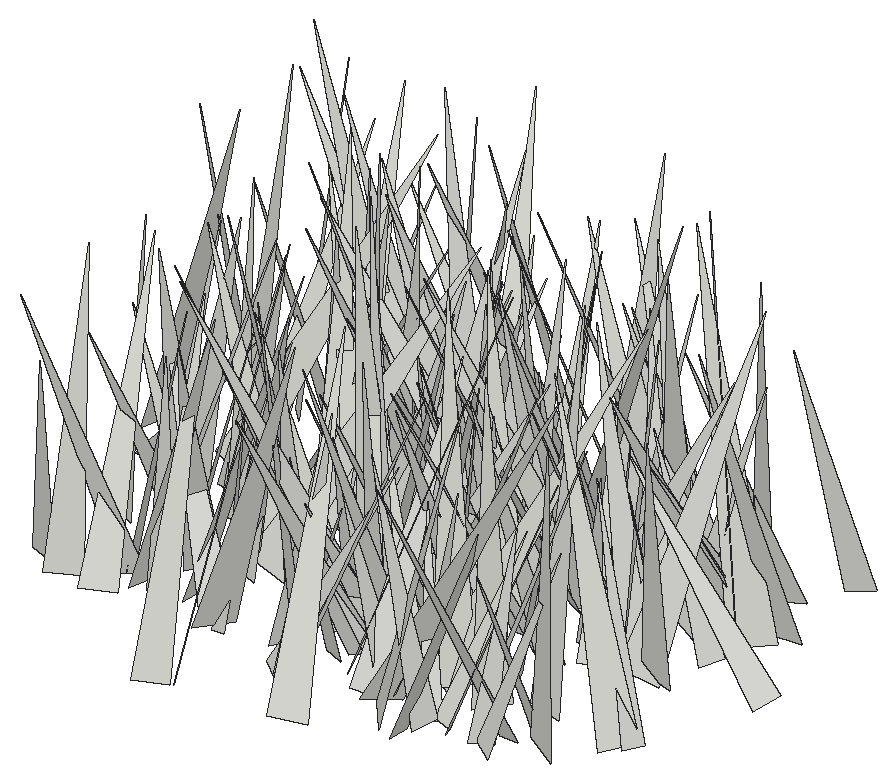
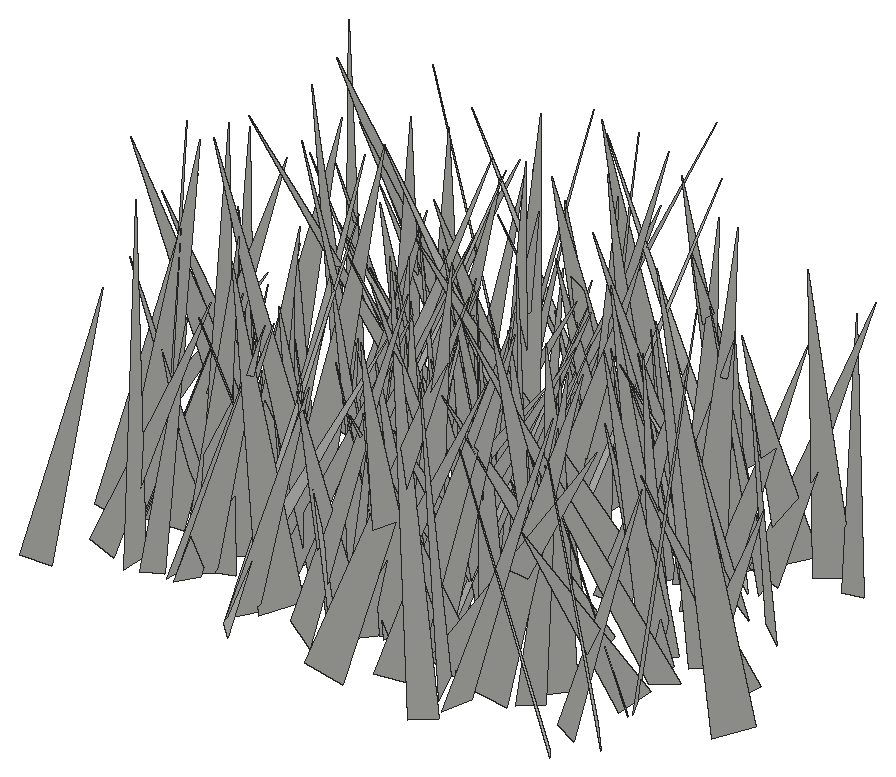
# SketchUp Ruby script. Lengths in inches.
U = 1.inch
M = Sketchup.active_model
def pt(a) = Geom::Point3d.new(a.map { |v| v * U })
def face(e, loops, mat)
  f = e.add_face(loops[0].map { |a| pt(a) })
  loops[1..].each { |l| e.add_face(l.map { |a| pt(a) }).erase! }
  f.material = f.back_material = mat if mat
  f
end
# faces: each face lists its corners as indices into pts; further lists are holes
def faces(e, pts, list, mat = nil) = list.each { |f| face(e, (f[0].is_a?(Array) ? f : [f]).map { |l| l.map { |i| pts[i] } }, mat) }
# xy, xz, yz: faces in a plane at the given z, y or x. An outline is a flat list of corners, or four numbers for a rectangle; further outlines are holes
def ring(l) = l.size == 4 ? [[l[0], l[1]], [l[2], l[1]], [l[2], l[3]], [l[0], l[3]]] : l.each_slice(2).to_a
def flat(e, list, mat, &to3) = list.each { |f| face(e, (f[0].is_a?(Array) ? f : [f]).map { |l| ring(l).map { |u, v| to3.(u, v) } }, mat) }
def xy(e, z, list, mat = nil) = flat(e, list, mat) { |x, y| [x, y, z] }
def xz(e, y, list, mat = nil) = flat(e, list, mat) { |x, z| [x, y, z] }
def yz(e, x, list, mat = nil) = flat(e, list, mat) { |y, z| [x, y, z] }
def lines(e, pts, list) = list.each { |a, b| e.add_line(pt(pts[a]), pt(pts[b])) }
# prism: a flat outline (further loops are holes) pulled along v
def prism(e, loops, v, mat = nil)
  f = face(e, loops, mat); d = Geom::Vector3d.new(v.map { |x| x * U })
  f.pushpull(f.normal.samedirection?(d) ? d.length : -d.length)
end
def box(e, o, s, mat = nil) = prism(e, [[o, [o[0] + s[0], o[1], o[2]], [o[0] + s[0], o[1] + s[1], o[2]], [o[0], o[1] + s[1], o[2]]]], [0, 0, s[2]], mat)
def at(x, y, z, deg = 0) = Geom::Transformation.translation(pt([x, y, z])) * Geom::Transformation.rotation(ORIGIN, Z_AXIS, deg.degrees)
def axes(o, x, y, z) = Geom::Transformation.new([*x, 0, *y, 0, *z, 0, *pt(o).to_a, 1])
def part(name) = M.definitions.add(name)
# library, detail: a bought-in or finely detailed component or shape, given as its bounding box
def library(name, o, s) = part(name).tap { |d| box(d.entities, o, s) }
def detail(e, o, s) = box(e.add_group.entities, o, s)
def put(e, d, t, mat = nil) = e.add_instance(d, t).tap { |i| i.material = mat if mat }
def group(e, t, mat = nil) = e.add_group.tap { |g| g.transformation = t; g.material = mat if mat }.entities
root = M.entities
c1 = part("fur_instance\#9")
p = [[0.8125,0,1.79],[0.67,-0.02,1.48],[0,-0.11,0],[0,0.11,0]]
faces(c1.entities,p,[[0,1,2,3]])
put(root,c1,axes([121.09,24.84,-27.1],[-5.92228,3.52878,0.304],[3.26745,5.67188,-2.1844],[1.36692,1.73077,6.53866]))
put(root,c1,axes([125.08,27.3125,-27.1],[6.15209,3.35933,0.33959],[3.37614,-6.1107,-0.71393],[0.04606,-0.78923,6.97306]))
put(root,c1,axes([133.24,29.44,-27.1],[-1.88046,-5.21634,0.33238],[-5.10911,1.75978,-1.28722],[-1.10347,0.74146,5.39346]))
put(root,c1,axes([128.65,27.92,-27.1],[5.36031,4.39922,1.5205],[4.6383,-5.24227,-1.18439],[-0.38885,-1.88772,6.83252]))
put(root,c1,axes([130.35,28.41,-27.1],[-5.09295,0.86723,1.4086],[1.03106,5.23004,0.50795],[1.29351,-0.75432,5.14123]))
put(root,c1,axes([121.52,25.7,-27.1],[6.37842,4.90538,1.53696],[4.59516,-6.53882,1.79932],[-2.30422,0.53885,7.84279]))
put(root,c1,axes([126.4375,25.72,-27.1],[-1.83957,6.80237,0.25254],[6.80704,1.83779,0.08208],[-0.01336,-0.2652,7.04624]))
put(root,c1,axes([112.64,29.51,-27.1],[-0.50328,-4.91347,1.0032],[-4.85841,0.72759,1.12622],[1.24277,0.85458,4.80907]))
put(root,c1,axes([120.26,29.36,-27.1],[6.42408,-3.63909,0.41323],[-3.66082,-6.40525,0.50369],[-0.11006,0.64215,7.36601]))
put(root,c1,axes([134.57,29.54,-27.1],[-2.31612,-6.1908,2.36322],[-6.27799,2.85121,1.3163],[2.12077,1.67923,6.47748]))
put(root,c1,axes([123.97,27.97,-27.1],[2.98745,4.37857,0.43851],[4.21633,-2.69647,-1.80015],[1.25963,-1.35874,4.98559]))
put(root,c1,axes([133,28.26,-27.1],[2.35379,3.88662,0.95748],[3.9563,-2.09005,-1.24191],[0.60851,-1.44527,4.3708]))
put(root,c1,axes([124.41,28.4,-27.1],[4.29417,-2.87763,1.75823],[-3.19183,-4.38696,0.6155],[-1.08829,1.5119,5.13243]))
put(root,c1,axes([124.15,29.3,-27.1],[-6.04607,-3.24149,2.31572],[-3.3744,6.40425,0.15438],[2.11738,0.95032,6.85845]))
put(root,c1,axes([125.6,31.08,-27.1],[1.43774,-5.64122,0.58152],[-5.34924,-1.54822,-1.79367],[-1.88339,0.09091,5.53834]))
put(root,c1,axes([133.97,30.2,-27.1],[-1.2303,-3.6424,0.32202],[-3.65502,1.23499,0.00478],[0.10759,0.30356,3.84457]))
put(root,c1,axes([132.68,28.6,-27.1],[-2.57998,2.99071,1.64125],[3.02202,2.95835,-0.64026],[1.58287,-0.77341,3.89753]))
put(root,c1,axes([126.14,31.38,-27.1],[-8.04638,-2.10125,0.20494],[-2.02323,7.90531,1.61682],[0.60315,-1.51404,8.15753]))
put(root,c1,axes([127.17,31.53,-27.1],[-6.19203,-3.31038,1.54754],[-2.85802,6.28451,2.00782],[2.2771,-1.114,6.72819]))
put(root,c1,axes([115.82,30.43,-27.1],[-0.4063,-5.76079,1.26429],[-5.69006,0.04941,-1.60344],[-1.5519,1.32705,5.54804]))
put(root,c1,axes([116.51,30.39,-27.1],[6.83641,-1.96558,0.32372],[-1.94381,-6.83529,-0.45298],[-0.43579,-0.34652,7.09893]))
put(root,c1,axes([117.53,29.95,-27.1],[1.49528,-4.80686,1.53266],[-5.04418,-1.45777,0.34917],[-0.10564,1.56838,5.02194]))
put(root,c1,axes([130.01,27.39,-27.1],[6.47636,2.00005,0.90058],[1.74291,-6.39683,1.67254],[-1.33173,1.35459,6.56857]))
put(root,c1,axes([127.65,29.78,-27.1],[-4.79801,0.15244,1.14259],[0.25589,4.91001,0.4195],[1.12396,-0.46714,4.78206]))
put(root,c1,axes([128.04,28.91,-27.1],[7.15691,-3.14413,0.26361],[-3.09126,-6.8566,2.14652],[0.63178,2.06831,7.5166]))
put(root,c1,axes([113.94,28.96,-27.1],[3.27303,-4.65782,3.06275],[-5.40234,-3.52629,0.41046],[-1.37496,2.76738,5.67799]))
put(root,c1,axes([130.34,28.77,-27.1],[-3.13044,2.30171,0.23571],[2.28042,3.13636,-0.34054],[0.39127,0.13578,3.8706]))
put(root,c1,axes([123.11,30.43,-27.1],[3.6641,-0.22277,0.06955],[-0.2117,-3.63329,-0.48425],[-0.09821,-0.47926,3.63879]))
put(root,c1,axes([117.4375,32.34,-27.1],[4.70982,-4.44224,0.12242],[-4.38661,-4.67586,-0.90827],[-0.71149,-0.57769,6.41023]))
put(root,c1,axes([125.21,32.375,-27.1],[3.98276,-1.20965,1.22676],[-0.42908,-3.68899,-2.24451],[-1.66855,-1.93873,3.5054]))
put(root,c1,axes([130.77,28.85,-27.1],[0.96645,3.75371,0.08435],[3.72936,-0.9496,-0.47076],[0.43512,-0.19848,3.84744]))
put(root,c1,axes([128.98,30.09,-27.1],[4.01363,-0.60213,1.19124],[-0.70216,-4.16285,0.26162],[-1.13516,0.446,4.0501]))
put(root,c1,axes([126.4,30.8125,-27.1],[5.75232,0.0292,2.58276],[0.25276,-6.28131,-0.49192],[-2.57052,-0.55229,5.73133]))
put(root,c1,axes([122.47,31.51,-27.1],[5.42089,-2.3865,1.81758],[-2.19868,-5.71457,-0.94576],[-2.04078,-0.18248,5.84696]))
put(root,c1,axes([128.19,29.92,-27.1],[5.44846,0.74036,0.07595],[0.73692,-5.44519,0.21553],[-0.10422,0.20337,5.4943]))
put(root,c1,axes([131.22,28.61,-27.1],[4.24517,2.47398,0.29086],[2.34061,-4.15824,1.20716],[-0.85248,0.90284,4.76286]))
put(root,c1,axes([124.87,30.25,-27.1],[-5.12266,-6.1706,2.10185],[-6.50165,4.64284,-2.21548],[-0.47189,3.01719,7.70776]))
put(root,c1,axes([122.875,29.83,-27.1],[5.08359,-0.28901,1.82683],[-0.68576,-5.25683,1.07667],[-1.71772,1.24337,4.97667]))
put(root,c1,axes([131.36,30.875,-27.1],[4.8811,-3.48072,2.77846],[-3.79933,-5.40519,-0.09683],[-2.32386,1.52607,5.99426]))
put(root,c1,axes([131.47,29.95,-27.1],[4.74716,3.3592,0.52437],[3.38285,-4.75689,-0.1518],[-0.33985,-0.42721,5.81349]))
put(root,c1,axes([119.93,29.96,-27.1],[-3.53792,4.34861,0.23075],[4.30519,3.44804,1.02808],[-0.65501,-0.82532,5.51093]))
put(root,c1,axes([127.45,28.9,-27.1],[-1.69129,6.09931,0.73665],[6.01995,1.79783,-1.06428],[1.22654,-0.41345,6.23934]))
put(root,c1,axes([124.03,32.61,-27.1],[4.34393,-1.36952,0.92271],[-1.07858,-4.31928,-1.3331],[-1.25046,-1.03195,4.35524]))
put(root,c1,axes([119.15,31.5,-27.1],[3.83115,1.46002,1.29175],[1.69697,-3.89964,-0.62537],[-0.95945,-1.06731,4.05194]))
put(root,c1,axes([115.32,31.03,-27.1],[5.01565,1.80166,1.23073],[1.89818,-5.12441,-0.23415],[-1.07592,-0.64182,5.32428]))
put(root,c1,axes([122.2,33.53,-27.1],[-5.96811,-4.81477,0.42538],[-4.75156,5.96808,0.88657],[0.88638,-0.42578,7.61672]))
put(root,c1,axes([115.61,28.8,-27.1],[-4.47188,4.60163,0.40246],[4.4512,4.44255,-1.33612],[1.23441,0.65071,6.27595]))
put(root,c1,axes([120.68,29.0625,-27.1],[2.07794,4.44656,0.23399],[4.16362,-2.03187,1.63715],[-1.57826,0.49406,4.62704]))
put(root,c1,axes([118.5,33.02,-27.1],[6.88515,-2.28469,0.18682],[-2.24647,-6.84269,-0.88939],[-0.45618,-0.78602,7.19959]))
put(root,c1,axes([115.79,33.53,-27.1],[0.74185,-5.118,0.35857],[-5.01336,-0.80012,-1.04825],[-1.09027,0.19676,5.06413]))
put(root,c1,axes([118.43,30.53,-27.1],[6.55283,1.12937,1.12544],[0.97488,-6.60494,0.95181],[-1.26162,0.76214,6.58096]))
put(root,c1,axes([128.43,33.79,-27.1],[1.50349,-5.86365,0.5049],[-5.82358,-1.55753,-0.74685],[-0.85041,0.2992,6.00709]))
put(root,c1,axes([123.91,32.0625,-27.1],[-5.32926,2.77314,1.19327],[2.9808,5.21718,1.1879],[0.47858,-1.6143,5.88899]))
put(root,c1,axes([136.55,31.375,-27.1],[-5.76808,3.66085,1.08427],[3.77252,5.76709,0.59739],[0.58783,-1.08949,6.80556]))
put(root,c1,axes([129.43,31.17,-27.1],[-5.69,4.35692,2.08043],[4.49689,5.95288,-0.16772],[1.75752,-1.1258,7.16454]))
put(root,c1,axes([115.99,33.63,-27.1],[4.78165,-4.93816,1.39024],[-4.88475,-4.96331,-0.82896],[-1.56762,0.40313,6.82367]))
put(root,c1,axes([125.73,30.17,-27.1],[6.75975,3.62956,0.52461],[3.54067,-6.74583,1.04905],[-0.95528,0.68056,7.60048]))
put(root,c1,axes([129.96,35.125,-27.1],[-4.86076,-4.47494,0.06756],[-4.36579,4.76306,1.38194],[0.98465,-0.972,6.46083]))
put(root,c1,axes([127.02,31.45,-27.1],[-4.60264,5.20733,0.96805],[5.29634,4.53648,0.77902],[0.04773,-1.24166,6.90606]))
put(root,c1,axes([127.35,33.32,-27.1],[-2.08811,-4.65792,0.59921],[-4.45757,1.75934,-1.85749],[-1.47829,1.27435,4.7546]))
put(root,c1,axes([124.63,33.22,-27.1],[-4.81324,5.46383,3.73935],[6.29264,5.21276,0.48307],[2.05886,-3.15867,7.26549]))
put(root,c1,axes([126.47,31.01,-27.1],[1.43872,7.93621,2.15807],[7.82752,-1.99366,2.11323],[-2.52399,-1.65906,7.7838]))
put(root,c1,axes([136.99,31.625,-27.1],[-4.67353,1.04438,0.03845],[1.02272,4.60667,-0.8165],[0.21505,0.78861,4.71868]))
put(root,c1,axes([133.02,31.72,-27.1],[2.04699,7.14679,2.15899],[7.40344,-2.23185,0.36858],[-0.96272,-1.9673,7.42502]))
put(root,c1,axes([118.97,32.75,-27.1],[1.57919,4.13225,1.33364],[4.34025,-1.54395,-0.35548],[-0.12772,-1.37428,4.40942]))
put(root,c1,axes([127.67,33.32,-27.1],[4.70905,2.28139,1.77217],[2.5251,-4.89691,-0.40574],[-1.40329,-1.15586,5.21682]))
put(root,c1,axes([128.81,31.12,-27.1],[2.72489,7.5123,0.23605],[7.26372,-2.56761,-2.13568],[1.931,-0.94238,7.70056]))
put(root,c1,axes([130.98,34.58,-27.1],[-0.18696,-5.47828,1.21386],[-5.53827,-0.01495,-0.92048],[-0.90141,1.22808,5.40363]))
put(root,c1,axes([116.23,30.89,-27.1],[4.52328,4.39752,0.22155],[4.10164,-4.32376,2.0806],[-1.60118,1.34692,5.95561]))
put(root,c1,axes([123.45,35.49,-27.1],[-3.4189,-2.83051,0.24342],[-2.77437,3.40847,0.66713],[0.61145,-0.36118,4.38812]))
put(root,c1,axes([134.63,35.83,-27.1],[-0.27546,-6.0552,1.07535],[-6.00995,0.49341,1.23885],[1.30474,0.99438,5.93351]))
put(root,c1,axes([125.12,34.48,-27.1],[2.82245,-3.27125,1.23973],[-3.47956,-2.78972,0.56063],[-0.36142,1.31172,4.28404]))
put(root,c1,axes([113.125,33.41,-27.1],[2.73063,4.59292,1.67983],[4.59916,-3.06583,0.90635],[-1.66266,-0.93747,5.2659]))
put(root,c1,axes([130.91,32.84,-27.1],[6.22186,3.72093,2.03459],[3.43335,-6.54009,1.46143],[-2.48938,0.27987,7.10078]))
put(root,c1,axes([127.45,35.09,-27.1],[-3.50463,1.38607,1.3282],[1.66931,3.56562,0.68373],[0.94799,-1.15452,3.70623]))
put(root,c1,axes([115.04,32.7,-27.1],[2.36342,5.34352,0.74133],[5.25737,-2.46286,0.99138],[-1.20944,-0.26392,5.75813]))
put(root,c1,axes([114.99,35.23,-27.1],[4.88196,1.64498,0.71636],[1.77456,-4.73338,-1.22423],[-0.26474,-1.39349,5.00407]))
put(root,c1,axes([128.9,35.49,-27.1],[-1.8038,-4.78632,0.84713],[-4.75617,1.55162,-1.36069],[-1.00264,1.25053,4.93062]))
put(root,c1,axes([131.8,37.64,-27.1],[-2.90473,-5.90083,0.221],[-5.68544,2.86131,1.67173],[1.5951,-0.54696,6.36102]))
put(root,c1,axes([125.07,33.88,-27.1],[2.90433,5.023,0.38727],[4.82562,-2.64532,-1.87916],[1.44702,-1.25991,5.48948]))
put(root,c1,axes([131.39,36.21,-27.1],[0.93641,-4.49496,0.58968],[-4.44892,-0.79539,1.00188],[0.87152,0.76939,4.48082]))
put(root,c1,axes([123.19,35.2,-27.1],[5.83146,1.27805,1.15338],[1.33487,-5.92923,-0.17895],[-1.08712,-0.42484,5.96719]))
put(root,c1,axes([118.87,35.04,-27.1],[-2.86629,5.19134,1.30889],[5.27356,2.48156,1.70596],[-0.92348,-1.94182,5.67938]))
put(root,c1,axes([128.82,38.29,-27.1],[-3.40543,-6.99905,0.02732],[-6.9991,3.40539,-0.01642],[-0.00281,0.03175,7.78353]))
put(root,c1,axes([126.48,36.89,-27.1],[-3.7934,-3.57067,0.95546],[-3.47781,3.9116,0.81037],[1.25196,0.04698,5.14615]))
put(root,c1,axes([119.21,33.55,-27.1],[-0.59602,7.49567,1.64856],[6.68012,1.32078,-3.59019],[3.77872,-1.15261,6.60687]))
put(root,c1,axes([134.82,36.22,-27.1],[-2.53419,-2.69204,0.92744],[-2.77792,2.61003,-0.01451],[0.6248,0.68554,3.69715]))
put(root,c1,axes([115.08,37.06,-27.1],[1.45023,-6.39796,1.08768],[-6.25164,-1.07813,1.99368],[1.74182,1.45734,6.24998]))
put(root,c1,axes([114.0625,35.53,-27.1],[-1.40668,3.30295,0.84871],[3.29754,1.08331,1.24951],[-0.86952,-1.23511,3.36556]))
put(root,c1,axes([129.87,38.51,-27.1],[2.52782,-6.77606,0.30453],[-6.73549,-2.54598,-0.74076],[-0.80053,0.02468,7.19418]))
put(root,c1,axes([113.36,36.58,-27.1],[2.93008,-5.46925,1.49234],[-5.65269,-2.69042,1.23848],[0.43226,1.89052,6.07982]))
put(root,c1,axes([138.625,36.93,-27.1],[-4.24155,2.82864,0.08548],[2.61337,3.85608,2.07369],[-1.08573,-1.76881,4.65744]))
put(root,c1,axes([116.31,35.5625,-27.1],[1.54209,5.92638,1.72605],[6.04197,-1.81335,0.82809],[-1.2633,-1.43843,6.06748]))
put(root,c1,axes([132.16,35.29,-27.1],[-1.31854,4.49628,0.43937],[4.51767,1.31381,0.11263],[0.01505,-0.45333,4.68427]))
put(root,c1,axes([114.54,37.66,-27.1],[1.31964,-4.20384,0.49444],[-3.9297,-1.02429,1.77946],[1.57296,0.96785,4.03079]))
put(root,c1,axes([111.18,37.04,-27.1],[2.58418,-3.37784,0.00054],[-2.92311,-2.23595,2.1316],[1.69269,1.29557,3.68023]))
put(root,c1,axes([127.53,36.53,-27.1],[-3.57367,4.96866,1.72232],[5.21894,3.60663,0.42422],[0.64547,-1.65218,6.10563]))
put(root,c1,axes([133.32,36.5,-27.1],[-5.60882,2.54428,1.1021],[2.59069,5.69507,0.03704],[0.9881,-0.48955,6.15881]))
put(root,c1,axes([132.29,38.31,-27.1],[0.84886,-4.32385,0.54485],[-4.30912,-0.7498,0.76315],[0.65118,0.6747,4.3398]))
put(root,c1,axes([132.6,36.36,-27.1],[-3.91577,-3.49387,3.17429],[-4.26524,4.38586,-0.43413],[2.02262,2.48468,5.2299]))
put(root,c1,axes([122.07,36.59,-27.1],[-0.00345,4.9845,1.60202],[5.18158,-0.22632,0.71534],[-0.75028,-1.58596,4.93291]))
put(root,c1,axes([134.37,40.42,-27.1],[4.00993,-5.51552,0.33203],[-5.14979,-3.87921,-2.24547],[-2.00271,-1.06842,6.43882]))
put(root,c1,axes([134.02,35.61,-27.1],[-1.22058,7.14872,1.6543],[7.02907,1.62036,-1.81584],[2.10547,-1.26529,7.02116]))
put(root,c1,axes([128.66,39.29,-27.1],[-6.87561,-0.89332,0.66489],[-0.69538,6.69239,1.80069],[0.86979,-1.71115,6.69549]))
put(root,c1,axes([131.08,36.83,-27.1],[0.63179,6.0642,2.01169],[5.81387,0.29266,-2.70812],[2.6496,-2.08816,5.46258]))
put(root,c1,axes([126.26,38.27,-27.1],[-2.43401,-4.94438,0.27236],[-4.40728,2.02468,-2.63096],[-2.25763,1.37813,4.84245]))
put(root,c1,axes([125.18,38.53,-27.1],[2.03296,-3.43324,0.36978],[-3.45285,-2.01606,0.26469],[0.04074,0.45292,3.9812]))
put(root,c1,axes([130.52,39.15,-27.1],[-1.29347,-4.18784,0.40951],[-4.17089,1.33267,0.45438],[0.55623,0.25449,4.35943]))
put(root,c1,axes([123.68,37.41,-27.1],[5.7925,1.49056,1.34896],[1.52882,-5.93778,-0.00376],[-1.30544,-0.3399,5.9812]))
put(root,c1,axes([120.92,37.8125,-27.1],[-2.66914,2.15187,1.53787],[2.38339,2.90414,0.07299],[1.14676,-1.02728,3.42776]))
put(root,c1,axes([131.25,37.58,-27.1],[-2.34168,-2.41248,1.9117],[-2.76899,2.70012,0.01564],[1.3444,1.35921,3.36204]))
put(root,c1,axes([135.36,38,-27.1],[-3.9914,1.89648,0.82188],[2.01712,3.964,0.64912],[0.45094,-0.94526,4.3711]))
put(root,c1,axes([122.61,39.7,-27.1],[-0.7364,-6.55979,0.93298],[-6.36781,0.44127,-1.92351],[-1.83094,1.10364,6.31453]))
put(root,c1,axes([123.43,37.85,-27.1],[-1.82115,-3.36265,1.61921],[-3.73204,1.65736,-0.7556],[0.03439,1.7865,3.74875]))
put(root,c1,axes([120.5,37.76,-27.1],[4.06784,5.47307,2.7985],[5.78633,-4.54195,0.47187],[-2.07475,-1.93641,6.80288]))
put(root,c1,axes([127.06,36.36,-27.1],[-6.05954,0.33778,0.89505],[0.02694,5.79744,-2.00555],[0.95629,1.97708,5.728]))
put(root,c1,axes([109.81,39.62,-27.1],[8.0282,-2.33719,0.44231],[-2.30718,-8.02996,-0.55383],[-0.57877,-0.40914,8.34313]))
put(root,c1,axes([125.32,38.08,-27.1],[-1.86227,-3.58892,1.59018],[-3.91628,1.57852,-1.02377],[-0.26793,1.87217,3.91156]))
put(root,c1,axes([134.66,41.36,-27.1],[-4.06772,-3.26977,0.32403],[-2.78571,3.7053,2.41936],[1.74246,-1.70943,4.62433]))
put(root,c1,axes([119.39,37.33,-27.1],[1.43263,3.39143,0.32506],[3.34277,-1.46736,0.57677],[-0.65831,-0.07043,3.63615]))
put(root,c1,axes([123.82,39.62,-27.1],[4.04014,-3.74392,1.13553],[-3.80741,-4.13804,-0.09691],[-0.90002,0.69913,5.50729]))
put(root,c1,axes([113.61,40.28,-27.1],[-6.01698,-4.0059,2.23214],[-3.85326,6.41302,1.12219],[2.48637,0.24439,7.14087]))
put(root,c1,axes([127.23,37.89,-27.1],[1.06492,5.99669,1.55027],[6.17359,-1.15473,0.22589],[-0.50038,-1.48458,6.08632]))
put(root,c1,axes([122.11,39.97,-27.1],[-5.99234,-4.15881,0.58341],[-4.19764,5.96205,-0.6148],[0.12593,0.83815,7.26814]))
put(root,c1,axes([119.22,37.2,-27.1],[-5.83364,4.02968,1.05878],[3.90844,5.92385,-1.01134],[1.44341,0.24573,7.01761]))
put(root,c1,axes([120.09,37.9,-27.1],[-5.57386,3.34507,0.61319],[3.34749,5.6042,-0.14346],[0.5998,-0.19191,6.49898]))
put(root,c1,axes([136.3125,40.92,-27.1],[-0.27695,-6.43694,1.01641],[-6.49492,0.18954,-0.56932],[-0.53231,1.03627,6.4177]))
put(root,c1,axes([118.17,39.37,-27.1],[5.45486,-2.53583,1.72286],[-2.73109,-5.61705,0.37948],[-1.39279,1.08278,6.00349]))
put(root,c1,axes([126.59,40.12,-27.1],[0.40641,-5.35004,1.66525],[-5.54368,-0.62666,-0.66032],[-0.81458,1.59547,5.32467]))
put(root,c1,axes([115.12,37.125,-27.1],[-7.30658,0.78889,2.52937],[0.00726,7.42557,-2.29501],[2.64953,2.15518,6.98151]))
put(root,c1,axes([126.48,40.625,-27.1],[4.42301,-0.66017,1.25029],[-0.31732,-4.46498,-1.23502],[-1.37781,-1.09094,4.29808]))
put(root,c1,axes([123.5,40.79,-27.1],[-6.69596,1.51903,0.23584],[1.52209,6.40398,1.96756],[-0.2152,-1.96993,6.57815]))
put(root,c1,axes([123.33,36.87,-27.1],[1.15921,7.66569,0.40932],[7.66684,-1.17697,0.3294],[-0.3873,-0.35503,7.74584]))
put(root,c1,axes([125.68,39.08,-27.1],[2.94995,3.39967,1.09614],[3.50655,-3.02709,-0.04841],[-0.68072,-0.86052,4.50085]))
put(root,c1,axes([116.93,37.8,-27.1],[5.85572,0.96623,0.0245],[0.91904,-5.61274,1.69591],[-0.29926,1.66948,5.68743]))
put(root,c1,axes([120.04,39.79,-27.1],[-0.77614,4.62516,2.62163],[4.88719,1.66369,-1.48826],[2.09294,-2.16967,4.44742]))
put(root,c1,axes([130.79,41.99,-27.1],[0.39282,-7.92697,1.06347],[-7.86049,-0.18606,1.51663],[1.47665,1.11832,7.79044]))
put(root,c1,axes([127.57,39.83,-27.1],[8.28106,0.30024,0.90595],[0.31898,-8.32832,-0.15571],[-0.89952,-0.18935,8.28504]))
put(root,c1,axes([133.2,39.24,-27.1],[2.00403,4.77087,1.2081],[4.88814,-1.77806,-1.08691],[0.57161,-1.52123,5.05925]))
put(root,c1,axes([116.21,41.15,-27.1],[5.02867,-2.50397,0.95955],[-2.41233,-5.11484,-0.70513],[-1.17101,-0.21602,5.57317]))
put(root,c1,axes([128.75,40.84,-27.1],[-2.94744,-5.34651,0.76174],[-5.29498,2.69026,-1.60576],[-1.06233,1.42484,5.89017]))
put(root,c1,axes([135.75,39.77,-27.1],[-4.55755,6.1935,2.40469],[6.62517,4.45559,1.08074],[0.49905,-2.58872,7.61332]))
put(root,c1,axes([135.03,39.68,-27.1],[-5.85102,-5.01294,3.05498],[-5.59861,6.06235,-0.77491],[1.76582,2.61061,7.66574]))
put(root,c1,axes([113.83,38.39,-27.1],[1.59933,7.72158,1.03232],[7.26868,-1.09996,-3.03359],[2.80263,-1.55359,7.2786]))
put(root,c1,axes([120.22,40.29,-27.1],[4.77754,4.17311,2.72058],[4.61145,-5.13068,-0.22808],[-1.8844,-1.97551,6.33938]))
put(root,c1,axes([119.35,37.45,-27.1],[-1.39232,7.88876,0.40308],[7.89477,1.37627,0.33483],[-0.26016,-0.45487,8.00369]))
put(root,c1,axes([118.83,41.48,-27.1],[0.4901,-6.09421,1.40714],[-6.12992,-0.18765,1.32232],[1.24239,1.47818,5.96918]))
put(root,c1,axes([120.79,38.41,-27.1],[-3.36626,3.2291,1.55087],[2.48228,3.63709,-2.18492],[2.58275,0.71309,4.12128]))
put(root,c1,axes([131.17,37.88,-27.1],[3.09687,5.17866,0.3937],[4.90573,-3.06729,1.75775],[-1.70508,0.58082,5.7723]))
put(root,c1,axes([132.82,39.97,-27.1],[-6.31107,2.62453,1.38258],[2.63294,6.45317,-0.23139],[1.36651,-0.31261,6.83112]))
put(root,c1,axes([122.08,41.1,-27.1],[2.26565,-5.57265,3.25786],[-5.77256,-3.29433,-1.62055],[-2.88887,2.21229,5.79322]))
put(root,c1,axes([113.57,40.8125,-27.1],[3.56732,3.05528,0.6125],[3.0981,-3.37772,-1.19517],[0.33415,-1.30074,4.54225]))
put(root,c1,axes([123.37,40.17,-27.1],[-7.4138,3.10521,1.79195],[3.13289,7.61249,-0.22981],[1.74312,-0.47482,8.03455]))
put(root,c1,axes([122.11,39.12,-27.1],[-0.74484,5.04348,0.31723],[4.84937,0.80355,-1.38926],[1.42161,-0.09859,4.90524]))
put(root,c1,axes([121.17,42.35,-27.1],[2.55159,-4.81811,0.15811],[-4.66384,-2.42197,1.46026],[1.21971,0.81832,5.25284]))
put(root,c1,axes([116.51,42.46,-27.1],[4.04472,-2.80495,1.23292],[-2.68281,-4.22845,-0.81868],[-1.47998,-0.00072,4.85358]))
put(root,c1,axes([130.94,40.68,-27.1],[-3.74669,3.50171,1.17991],[3.59906,3.83892,0.03541],[0.8372,-0.8322,5.12819]))
put(root,c1,axes([129.78,41.62,-27.1],[-5.18196,-4.15409,0.26027],[-4.02731,4.89921,-1.98883],[-1.05116,1.70828,6.3367]))
put(root,c1,axes([125.33,41.33,-27.1],[-5.00491,-0.78513,1.46412],[-0.94309,5.16869,-0.45214],[1.36772,0.69095,5.0459]))
put(root,c1,axes([117.93,40.13,-27.1],[-5.27031,-0.93158,1.82448],[-1.52104,5.15288,-1.7627],[1.37223,2.13373,5.05341]))
put(root,c1,axes([121.33,43.98,-27.1],[3.93068,-5.30389,1.53813],[-4.85639,-4.21869,-2.1367],[-2.62918,-0.13704,6.24628]))
put(root,c1,axes([132.51,43.35,-27.1],[3.93846,-2.19121,0.70559],[-1.95473,-3.92185,-1.26841],[-1.21585,-0.79274,4.32481]))
put(root,c1,axes([134.93,43.1,-27.1],[-0.6126,-5.21006,0.97224],[-5.10965,0.32064,-1.50131],[-1.40764,1.1035,5.02654]))
put(root,c1,axes([127.97,44.95,-27.1],[-5.57338,-5.53642,0.81265],[-5.27737,5.58191,1.83481],[1.86058,-0.75178,7.63858]))
put(root,c1,axes([124.06,42.42,-27.1],[-6.12139,2.10353,0.29479],[2.12072,6.0019,1.20952],[-0.1196,-1.23917,6.35872]))
put(root,c1,axes([131.29,42.95,-27.1],[-5.2528,1.04607,1.18822],[1.28573,5.22141,1.0871],[0.92359,-1.31932,5.24446]))
put(root,c1,axes([131.82,42.88,-27.1],[-5.37487,-0.5228,0.79074],[-0.44432,5.41107,0.55741],[0.83736,-0.48456,5.37139]))
put(root,c1,axes([114.31,43.25,-27.1],[-1.82389,-4.57282,0.8897],[-4.65371,1.74485,-0.5721],[-0.21262,1.03617,4.88978]))
put(root,c1,axes([133.42,43.16,-27.1],[6.36794,0.62079,2.33056],[0.97414,-6.68136,-0.88201],[-2.20634,-1.15823,6.33704]))
put(root,c1,axes([123.21,41.38,-27.1],[-4.28711,2.60894,1.39768],[2.40918,4.50508,-1.01958],[1.71929,0.19268,4.91389]))
put(root,c1,axes([119.54,42.01,-27.1],[3.95352,-1.35205,0.74696],[-1.51739,-3.78343,1.18299],[-0.28899,1.3689,4.00736]))
put(root,c1,axes([118.78,45.56,-27.1],[8.12463,-0.31909,0.21051],[-0.21684,-7.53553,-3.0536],[-0.31483,-3.04462,7.53571]))
put(root,c1,axes([123.47,45.2,-27.1],[0.28426,-7.43419,0.75555],[-7.30944,-0.43371,-1.51752],[-1.55247,0.68085,7.28321]))
put(root,c1,axes([125.8,43.5625,-27.1],[-3.53449,-6.31522,1.62159],[-6.50822,3.306,-1.31053],[-0.39309,2.04757,7.11738]))
put(root,c1,axes([125.5,41.51,-27.1],[-4.48164,3.41054,1.04148],[3.17852,4.57879,-1.31654],[1.61662,0.45221,5.47573]))
put(root,c1,axes([131.28,42.4375,-27.1],[-5.13567,3.95215,0.39173],[3.97037,5.09374,0.66187],[-0.09557,-0.76314,6.44644]))
put(root,c1,axes([123.96,43.88,-27.1],[4.93042,2.67254,1.54888],[2.99605,-4.84755,-1.1728],[-0.75178,-1.79146,5.48417]))
put(root,c1,axes([118.12,42.97,-27.1],[-2.53782,7.33959,2.16761],[7.45924,1.86167,2.42953],[-1.71111,-2.77006,7.37615]))
put(root,c1,axes([113.84,40.05,-27.1],[-4.95607,3.58078,0.35964],[3.00453,4.45388,-2.94106],[1.98095,2.2034,5.36049]))
put(root,c1,axes([120.14,42.46,-27.1],[-2.8355,7.09509,0.7949],[6.33308,2.10473,3.80453],[-3.2961,-2.05963,6.62616]))
put(root,c1,axes([127.45,42.54,-27.1],[5.828,-3.21448,3.45143],[-4.0564,-6.21538,1.06086],[-2.40642,2.69201,6.57061]))
put(root,c1,axes([122.92,41.47,-27.1],[-3.64093,6.72533,0.73654],[6.73348,3.68347,-0.34805],[0.65778,-0.48058,7.63972]))
put(root,c1,axes([118.45,44.11,-27.1],[-6.63907,0.80935,0.83748],[0.8673,6.67065,0.42894],[0.7773,-0.53025,6.67446]))
put(root,c1,axes([136.18,45.17,-27.1],[1.56838,-4.91392,1.31708],[-4.91027,-1.82266,-0.95305],[-1.33063,0.93404,5.06933]))
put(root,c1,axes([119.55,43.38,-27.1],[-5.60874,-1.91132,2.91151],[-2.48414,6.06379,-0.80475],[2.44113,1.77916,5.87056]))
put(root,c1,axes([128.22,43.74,-27.1],[-5.4054,2.23783,0.44972],[2.26041,5.40869,0.2551],[0.31726,-0.40826,5.84475]))
put(root,c1,axes([113.28,42.71,-27.1],[4.45887,4.52554,1.75159],[4.30275,-4.78695,1.41478],[-2.24387,-0.18639,6.19358]))
put(root,c1,axes([113.875,44.71,-27.1],[4.52674,3.32324,0.78926],[3.39525,-4.2348,-1.64226],[0.37301,-1.78348,5.37013]))
